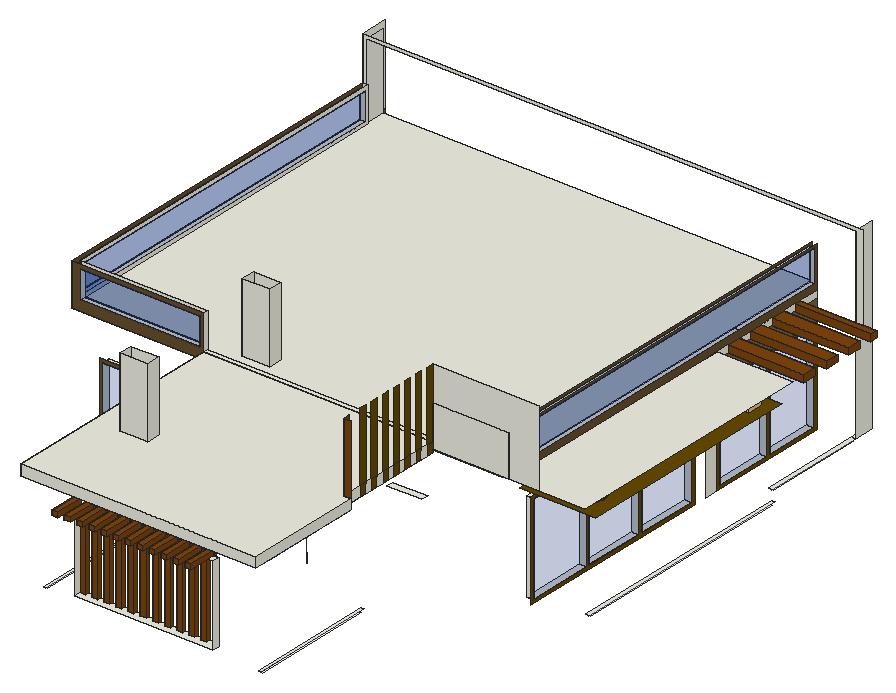
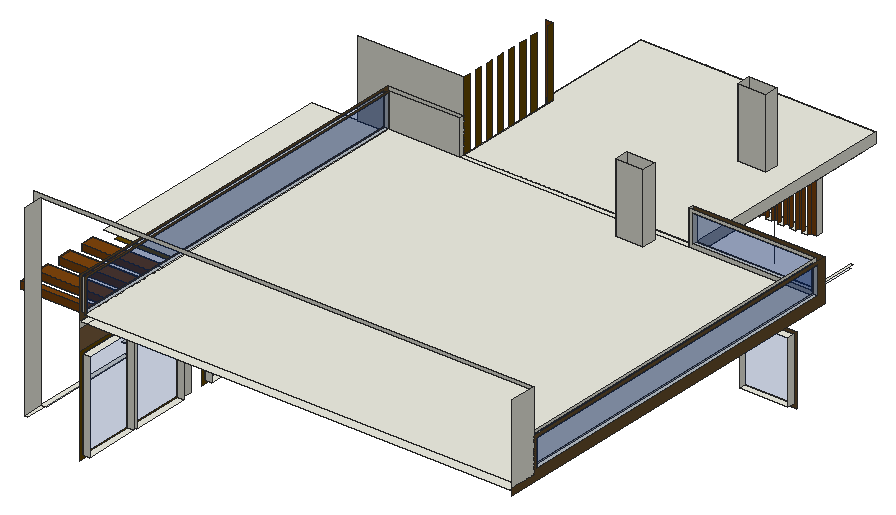
# SketchUp Ruby script. Lengths in inches.
U = 1.inch
M = Sketchup.active_model
def pt(a) = Geom::Point3d.new(a.map { |v| v * U })
def face(e, loops, mat)
  f = e.add_face(loops[0].map { |a| pt(a) })
  loops[1..].each { |l| e.add_face(l.map { |a| pt(a) }).erase! }
  f.material = f.back_material = mat if mat
  f
end
# faces: each face lists its corners as indices into pts; further lists are holes
def faces(e, pts, list, mat = nil) = list.each { |f| face(e, (f[0].is_a?(Array) ? f : [f]).map { |l| l.map { |i| pts[i] } }, mat) }
# xy, xz, yz: faces in a plane at the given z, y or x. An outline is a flat list of corners, or four numbers for a rectangle; further outlines are holes
def ring(l) = l.size == 4 ? [[l[0], l[1]], [l[2], l[1]], [l[2], l[3]], [l[0], l[3]]] : l.each_slice(2).to_a
def flat(e, list, mat, &to3) = list.each { |f| face(e, (f[0].is_a?(Array) ? f : [f]).map { |l| ring(l).map { |u, v| to3.(u, v) } }, mat) }
def xy(e, z, list, mat = nil) = flat(e, list, mat) { |x, y| [x, y, z] }
def xz(e, y, list, mat = nil) = flat(e, list, mat) { |x, z| [x, y, z] }
def yz(e, x, list, mat = nil) = flat(e, list, mat) { |y, z| [x, y, z] }
def lines(e, pts, list) = list.each { |a, b| e.add_line(pt(pts[a]), pt(pts[b])) }
# prism: a flat outline (further loops are holes) pulled along v
def prism(e, loops, v, mat = nil)
  f = face(e, loops, mat); d = Geom::Vector3d.new(v.map { |x| x * U })
  f.pushpull(f.normal.samedirection?(d) ? d.length : -d.length)
end
def box(e, o, s, mat = nil) = prism(e, [[o, [o[0] + s[0], o[1], o[2]], [o[0] + s[0], o[1] + s[1], o[2]], [o[0], o[1] + s[1], o[2]]]], [0, 0, s[2]], mat)
def at(x, y, z, deg = 0) = Geom::Transformation.translation(pt([x, y, z])) * Geom::Transformation.rotation(ORIGIN, Z_AXIS, deg.degrees)
def axes(o, x, y, z) = Geom::Transformation.new([*x, 0, *y, 0, *z, 0, *pt(o).to_a, 1])
def part(name) = M.definitions.add(name)
# library, detail: a bought-in or finely detailed component or shape, given as its bounding box
def library(name, o, s) = part(name).tap { |d| box(d.entities, o, s) }
def detail(e, o, s) = box(e.add_group.entities, o, s)
def put(e, d, t, mat = nil) = e.add_instance(d, t).tap { |i| i.material = mat if mat }
def group(e, t, mat = nil) = e.add_group.tap { |g| g.transformation = t; g.material = mat if mat }.entities
root = M.entities
M.materials.add("C08_Toffee_Ember").color = [127, 69, 12]
M.materials.add("D01_Frost_White").color = [238, 238, 227]
M.materials.add("D08_Bronzed_Mustard").color = [102, 74, 0]
M.materials.add("Glass_Basic_01").color = [161, 173, 186]
M.materials["Glass_Basic_01"].alpha = 0.25
M.materials.add("Glass_Sky Reflection_01").color = [0, 46, 142]
M.materials["Glass_Sky Reflection_01"].alpha = 0.25
M.materials.add("Plywood_01_1K").color = [125, 96, 64]
M.materials.add("Wood_Veneer_15_1K").color = [103, 79, 44]
c1 = part("Group71\#2")
p = [[0,0,0],[0,0,-29.19],[-0.46,0,-29.19],[3,-91.5,0],[-3,-91.5,0],[3,91.5,0],
  [3,0,0],[-3,91.5,0],[0.46,0,-29.19],[-3,0,0],[0,0,-47.25]]
lines(c1.entities,p,[[0,1],[1,2],[3,4],[5,6],[7,5],[1,8],[9,0],[0,6],[8,10],[4,9],[6,3],[2,10],
  [9,7]])
c2 = part("Rectangle Light")
put(c2.entities,c1,at(0,0,0))
c3 = part("Group73\#1")
p = [[0,0,0],[0,0,-14.36],[-0.46,0,-14.36],[3,-43.5,0],[-3,-43.5,0],[3,43.5,0],
  [3,0,0],[-3,43.5,0],[0.46,0,-14.36],[-3,0,0],[0,0,-23.25]]
lines(c3.entities,p,[[0,1],[1,2],[3,4],[5,6],[7,5],[1,8],[9,0],[0,6],[8,10],[4,9],[6,3],[2,10],
  [9,7]])
c4 = part("Rectangle Light\#1")
put(c4.entities,c3,at(0,0,0))
c5 = library("Sphere Light\#17",[-6.75,-6.75,-6.75],[13.5,13.5,13.5])
c6 = library("Sphere Light\#18",[-6.55,-6.55,-6.55],[13.1,13.1,13.1])
c7 = library("Sphere Light\#15",[-5.37,-5.37,-5.37],[10.74,10.74,10.74])
c8 = library("Sphere Light\#16",[-5.33,-5.33,-5.33],[10.66,10.66,10.66])
xy(root,165,[[376,388,382,445.01],[376,448.01,382,502.01],[376,505.01,382,559.02],[376,589,382,640],[376,643,382,691]],"D01_Frost_White")
xy(root,175,[[126,180,128,359],[312,180,314,287]],"Glass_Basic_01")
xy(root,177,[[126,178,128,361],[312,178,314,289]],"D01_Frost_White")
xy(root,178,[[439,375,442,572.02],[427,588,430,674]],"Glass_Basic_01")
xy(root,180,[[439,373,442,574.02],[427,586,430,676],[427,676,430,694]],"D01_Frost_White")
xy(root,183,[[31,361,73,367]],"D01_Frost_White")
xy(root,186,[[160,169,280,169,280,175,274.78,175,274.78,178,269.57,178,269.57,175,264.35,175,264.35,178,259.13,178,259.13,175,253.91,175,253.91,178,248.7,178,248.7,175,243.48,175,243.48,178,238.26,178,238.26,175,233.04,175,233.04,178,227.83,178,227.83,175,222.61,175,222.61,178,217.39,178,217.39,175,212.17,175,212.17,178,206.96,178,206.96,175,201.74,175,201.74,178,196.52,178,196.52,175,191.3,175,191.3,178,186.09,178,186.09,175,180.87,175,180.87,178,175.65,178,175.65,175,170.43,175,170.43,178,165.22,178,165.22,175,160,175]],"D01_Frost_White")
xy(root,218,[[138,361,158,367]],"D01_Frost_White")
xy(root,228,[[277,361,307,367]],"D01_Frost_White")
xy(root,237,[[31,361,73,367]],"D01_Frost_White")
xy(root,238,[[138,361,158,367]],"D01_Frost_White")
xy(root,243,[[376,388,382,445.01],[376,448.01,382,502.01],[376,505.01,382,559.02],[376,589,382,640],[376,643,382,691]],"D01_Frost_White")
xy(root,255,[[160,169,160,175,165.22,175,165.22,178,170.43,178,170.43,175,175.65,175,175.65,178,180.87,178,180.87,175,186.09,175,186.09,178,191.3,178,191.3,175,196.52,175,196.52,178,201.74,178,201.74,175,206.96,175,206.96,178,212.17,178,212.17,175,217.39,175,217.39,178,222.61,178,222.61,175,227.83,175,227.83,178,233.04,178,233.04,175,238.26,175,238.26,178,243.48,178,243.48,175,248.7,175,248.7,178,253.91,178,253.91,175,259.13,175,259.13,178,264.35,178,264.35,175,269.57,175,269.57,178,274.78,178,274.78,175,280,175,280,169]],"D01_Frost_White")
xy(root,258,[[[382,373,448,574.02],[429.95,390.2,431.52,390.3125,432.99,390.83,434.29,391.71,435.3125,392.9,435.99,394.31,436.28,395.85,436.17,397.41,435.65,398.89,434.77,400.18,433.58,401.2,432.17,401.88,430.63,402.18,429.07,402.06,427.59,401.54,426.3,400.66,425.28,399.48,424.6,398.06,424.3,396.53,424.42,394.96,424.9375,393.49,425.82,392.19,427,391.17,428.42,390.49],[388.9375,390.2,390.5,390.3125,391.98,390.83,393.27,391.71,394.3,392.9,394.98,394.31,395.27,395.85,395.15,397.41,394.64,398.89,393.75,400.18,392.57,401.2,391.16,401.88,389.62,402.18,388.06,402.06,386.58,401.54,385.28,400.66,384.26,399.48,383.58,398.06,383.29,396.53,383.4,394.96,383.92,393.49,384.8,392.19,385.99,391.17,387.4,390.49],[388.9375,551.54,390.5,551.66,391.98,552.17,393.27,553.06,394.3,554.24,394.98,555.65,395.27,557.19,395.15,558.75,394.64,560.23,393.75,561.53,392.57,562.55,391.16,563.23,389.62,563.52,388.06,563.41,386.58,562.89,385.28,562.01,384.26,560.82,383.58,559.41,383.29,557.87,383.4,556.31,383.92,554.83,384.8,553.54,385.99,552.51,387.4,551.83],[429.95,551.54,431.52,551.66,432.99,552.17,434.29,553.06,435.3125,554.24,435.99,555.65,436.28,557.19,436.17,558.75,435.65,560.23,434.77,561.53,433.58,562.55,432.17,563.23,430.63,563.52,429.07,563.41,427.59,562.89,426.3,562.01,425.28,560.82,424.6,559.41,424.3,557.87,424.42,556.31,424.9375,554.83,425.82,553.54,427,552.51,428.42,551.83]]],"D08_Bronzed_Mustard")
xy(root,259,[[160,145,165.22,169],[170.43,145,175.65,169],[180.87,145,186.09,169],[191.3,145,196.52,169],[201.74,145,206.96,169],
  [212.17,145,217.39,169],[222.61,145,227.83,169],[233.04,145,238.26,169],[243.48,145,248.7,169],[253.91,145,259.13,169],
  [264.35,145,269.57,169],[274.78,145,280,169]],"D08_Bronzed_Mustard")
xy(root,261,[[388.9375,390.2,387.4,390.49,385.99,391.17,384.8,392.19,383.92,393.49,383.4,394.96,383.29,396.53,383.58,398.06,384.26,399.48,385.28,400.66,386.58,401.54,388.06,402.06,389.62,402.18,391.16,401.88,392.57,401.2,393.75,400.18,394.64,398.89,395.15,397.41,395.27,395.85,394.98,394.31,394.3,392.9,393.27,391.71,391.98,390.83,390.5,390.3125],[429.95,390.2,428.42,390.49,427,391.17,425.82,392.19,424.9375,393.49,424.42,394.96,424.3,396.53,424.6,398.06,425.28,399.48,426.3,400.66,427.59,401.54,429.07,402.06,430.63,402.18,432.17,401.88,433.58,401.2,434.77,400.18,435.65,398.89,436.17,397.41,436.28,395.85,435.99,394.31,435.3125,392.9,434.29,391.71,432.99,390.83,431.52,390.3125],[388.9375,551.54,387.4,551.83,385.99,552.51,384.8,553.54,383.92,554.83,383.4,556.31,383.29,557.87,383.58,559.41,384.26,560.82,385.28,562.01,386.58,562.89,388.06,563.41,389.62,563.52,391.16,563.23,392.57,562.55,393.75,561.53,394.64,560.23,395.15,558.75,395.27,557.19,394.98,555.65,394.3,554.24,393.27,553.06,391.98,552.17,390.5,551.66],[429.95,551.54,428.42,551.83,427,552.51,425.82,553.54,424.9375,554.83,424.42,556.31,424.3,557.87,424.6,559.41,425.28,560.82,426.3,562.01,427.59,562.89,429.07,563.41,430.63,563.52,432.17,563.23,433.58,562.55,434.77,561.53,435.65,560.23,436.17,558.75,436.28,557.19,435.99,555.65,435.3125,554.24,434.29,553.06,432.99,552.17,431.52,551.66]],"D08_Bronzed_Mustard")
xy(root,263,[[160,145,165.22,169],[170.43,145,175.65,169],[180.87,145,186.09,169],[191.3,145,196.52,169],[201.74,145,206.96,169],
  [212.17,145,217.39,169],[222.61,145,227.83,169],[233.04,145,238.26,169],[243.48,145,248.7,169],[253.91,145,259.13,169],
  [264.35,145,269.57,169],[274.78,145,280,169]],"C08_Toffee_Ember")
xy(root,264,[[382,598,448,610],[382,622,448,634],[382,646,448,658],[382,670,448,676.01]],"C08_Toffee_Ember")
xy(root,267,[[118,163,118,361,316,361,316,178,322,178,322,163],[124,169,124,178,322,178,322,265,316,265,316,169],[316,178,322,265]],"D01_Frost_White")
xy(root,270,[[382,598,448,610],[382,622,448,634],[382,646,448,658],[382,670,448,670,448,676.01,436,676.01,436,676,430,676,430,676.01,382,676.01]],"C08_Toffee_Ember")
xy(root,270,[[124,169,316,178],[4,361,10,694],[10,361,376,367],[376,361,382,694],[382,361,448,586],
  [10,367,376,694],[430,676,436,676.01]],"D01_Frost_White")
xy(root,276,[[[118,163,322,163,322,265,316,265,316,361,118,361],[142,241,166,253]],[118,361,316,365.5],[[8.5,365.5,377.5,365.5,377.5,694,7,694,7,676.01,8.5,676.01],[142,373,166,385]],[377.5,365.5,382,610],[377.5,610,382,692]],"D01_Frost_White")
xy(root,279,[[11.5,361,115,365.5],[4,368.5,8.5,673.01]],"D01_Frost_White")
xz(root,145,[[160,259,165.22,263],[170.43,259,175.65,263],[180.87,259,186.09,263],[191.3,259,196.52,263],[201.74,259,206.96,263],
  [212.17,259,217.39,263],[222.61,259,227.83,263],[233.04,259,238.26,263],[243.48,259,248.7,263],[253.91,259,259.13,263],
  [264.35,259,269.57,263],[274.78,259,280,263]],"C08_Toffee_Ember")
xz(root,163,[[118,267,322,276]],"D01_Frost_White")
xz(root,169,[[124,267,316,270]],"D01_Frost_White")
xz(root,175,[[160,186,165.22,255],[170.43,186,175.65,255],[180.87,186,186.09,255],[191.3,186,196.52,255],[201.74,186,206.96,255],
  [212.17,186,217.39,255],[222.61,186,227.83,255],[233.04,186,238.26,255],[243.48,186,248.7,255],[253.91,186,259.13,255],
  [264.35,186,269.57,255],[274.78,186,280,255]],"C08_Toffee_Ember")
xz(root,178,[[124,267,316,270]],"D01_Frost_White")
xz(root,241,[[142,276,166,336]],"D01_Frost_White")
xz(root,253,[[142,276,166,336]],"D01_Frost_White")
xz(root,265,[[316,276,322,336]],"C08_Toffee_Ember")
xz(root,265,[[316,267,322,276]],"D08_Bronzed_Mustard")
xz(root,361,[[118,267,316,270],[118,270,316,276],[316,270,382,306],[382,270,382,306,316,306,316,336,408,336,408,270]],"D01_Frost_White")
xz(root,361,[[31,183,73,237],[138,218,158,238],[11.5,279,115,303]],"Glass_Sky Reflection_01")
xz(root,361,[[[28,180,76,240],[31,183,73,237]],[[136,216,160,240],[138,218,158,238]],[[4,270,118,306],[11.5,279,115,303]]],"Wood_Veneer_15_1K")
xz(root,365.5,[[[8.5,276,118,306],[11.5,279,115,303]],[316,276,377.5,306],[377.5,276,382,304]],"D01_Frost_White")
xz(root,365.5,[[11.5,279,115,303]],"Glass_Sky Reflection_01")
xz(root,368.5,[[4,279,8.5,303]],"D01_Frost_White")
xz(root,373,[[142,276,166,336]],"D01_Frost_White")
xz(root,385,[[142,276,166,336]],"D01_Frost_White")
xz(root,388,[[376,165,382,243]],"D01_Frost_White")
xz(root,445.01,[[376,165,382,243]],"D01_Frost_White")
xz(root,448.01,[[376,165,382,243]],"D01_Frost_White")
xz(root,502.01,[[376,165,382,243]],"D01_Frost_White")
xz(root,505.01,[[376,165,382,243]],"D01_Frost_White")
xz(root,559.02,[[376,165,382,243]],"D01_Frost_White")
xz(root,589,[[376,165,382,243]],"D01_Frost_White")
xz(root,598,[[382,264,448,270]],"C08_Toffee_Ember")
xz(root,610,[[382,264,448,270]],"C08_Toffee_Ember")
xz(root,622,[[382,264,448,270]],"C08_Toffee_Ember")
xz(root,634,[[382,264,448,270]],"C08_Toffee_Ember")
xz(root,640,[[376,165,382,243]],"D01_Frost_White")
xz(root,643,[[376,165,382,243]],"D01_Frost_White")
xz(root,646,[[382,264,448,270]],"C08_Toffee_Ember")
xz(root,658,[[382,264,448,270]],"C08_Toffee_Ember")
xz(root,670,[[382,264,448,270]],"C08_Toffee_Ember")
xz(root,673.01,[[4,279,8.5,303]],"D01_Frost_White")
xz(root,676.01,[[382,264,448,270]],"C08_Toffee_Ember")
xz(root,676.01,[[430,270,436,270,436,344,4,344,4,306,7,306,7,341,430,341],[7,276,8.5,306]],"D01_Frost_White")
xz(root,691,[[376,165,382,243]],"D01_Frost_White")
xz(root,692,[[377.5,276,382,304]],"D01_Frost_White")
yz(root,4,[[676.01,276,700,344]],"D01_Frost_White")
yz(root,4,[[368.5,279,673.01,303]],"Glass_Sky Reflection_01")
yz(root,4,[[[361,270,361,306,676.01,306,676.01,276,700,276,700,270],[368.5,279,673.01,303]]],"Wood_Veneer_15_1K")
yz(root,7,[[676.01,276,694,341]],"D01_Frost_White")
yz(root,8.5,[[[365.5,276,676.01,306],[368.5,279,673.01,303]]],"D01_Frost_White")
yz(root,8.5,[[368.5,279,673.01,303]],"Glass_Sky Reflection_01")
yz(root,11.5,[[361,279,365.5,303]],"D01_Frost_White")
yz(root,31,[[361,183,367,237]],"D01_Frost_White")
yz(root,73,[[361,183,367,237]],"D01_Frost_White")
yz(root,115,[[361,279,365.5,303]],"D01_Frost_White")
yz(root,118,[[163,267,361,276],[361,276,365.5,306]],"D01_Frost_White")
yz(root,124,[[169,267,178,270]],"D01_Frost_White")
yz(root,138,[[361,218,367,238]],"D01_Frost_White")
yz(root,142,[[241,276,253,336],[373,276,385,336]],"D01_Frost_White")
yz(root,158,[[361,218,367,238]],"D01_Frost_White")
yz(root,160,[[145,259,169,263]],"C08_Toffee_Ember")
yz(root,160,[[169,186,175,255]],"D01_Frost_White")
yz(root,165.22,[[175,186,178,255],[145,259,169,263]],"C08_Toffee_Ember")
yz(root,166,[[241,276,253,336],[373,276,385,336]],"D01_Frost_White")
yz(root,170.43,[[175,186,178,255],[145,259,169,263]],"C08_Toffee_Ember")
yz(root,175.65,[[175,186,178,255],[145,259,169,263]],"C08_Toffee_Ember")
yz(root,180.87,[[175,186,178,255],[145,259,169,263]],"C08_Toffee_Ember")
yz(root,186.09,[[175,186,178,255],[145,259,169,263]],"C08_Toffee_Ember")
yz(root,191.3,[[175,186,178,255],[145,259,169,263]],"C08_Toffee_Ember")
yz(root,196.52,[[175,186,178,255],[145,259,169,263]],"C08_Toffee_Ember")
yz(root,201.74,[[175,186,178,255],[145,259,169,263]],"C08_Toffee_Ember")
yz(root,206.96,[[175,186,178,255],[145,259,169,263]],"C08_Toffee_Ember")
yz(root,212.17,[[175,186,178,255],[145,259,169,263]],"C08_Toffee_Ember")
yz(root,217.39,[[175,186,178,255],[145,259,169,263]],"C08_Toffee_Ember")
yz(root,222.61,[[175,186,178,255],[145,259,169,263]],"C08_Toffee_Ember")
yz(root,227.83,[[175,186,178,255],[145,259,169,263]],"C08_Toffee_Ember")
yz(root,233.04,[[175,186,178,255],[145,259,169,263]],"C08_Toffee_Ember")
yz(root,238.26,[[175,186,178,255],[145,259,169,263]],"C08_Toffee_Ember")
yz(root,243.48,[[175,186,178,255],[145,259,169,263]],"C08_Toffee_Ember")
yz(root,248.7,[[175,186,178,255],[145,259,169,263]],"C08_Toffee_Ember")
yz(root,253.91,[[175,186,178,255],[145,259,169,263]],"C08_Toffee_Ember")
yz(root,259.13,[[175,186,178,255],[145,259,169,263]],"C08_Toffee_Ember")
yz(root,264.35,[[175,186,178,255],[145,259,169,263]],"C08_Toffee_Ember")
yz(root,269.57,[[175,186,178,255],[145,259,169,263]],"C08_Toffee_Ember")
yz(root,274.78,[[175,186,178,255],[145,259,169,263]],"C08_Toffee_Ember")
yz(root,280,[[145,259,169,263]],"C08_Toffee_Ember")
yz(root,280,[[169,186,175,255]],"D01_Frost_White")
yz(root,316,[[169,267,178,270],[271,267,283,276],[289,267,295,276],[301,267,307,276],[313,267,319,276],
  [325,267,331,276],[337,267,343,276],[349,267,355,276],[361,276,365.5,306]],"D01_Frost_White")
yz(root,316,[[265,267,271,276],[283,267,289,276],[295,267,301,276],[307,267,313,276],[319,267,325,276],
  [331,267,337,276],[343,267,349,276],[355,267,361,276],[265,276,271,336],[283,276,289,336],
  [295,276,301,336],[307,276,313,336],[319,276,325,336],[331,276,337,336],[343,276,349,336],
  [355,276,361,336]],"D08_Bronzed_Mustard")
yz(root,322,[[163,267,265,276]],"D01_Frost_White")
yz(root,377.5,[[365.5,276,692,304]],"Glass_Sky Reflection_01")
yz(root,377.5,[[692,276,692,304,365.5,304,365.5,306,694,306,694,276]],"Wood_Veneer_15_1K")
yz(root,382,[[574.02,162,586,246],[574.02,246,586,270],[586,264,598,270],[610,264,622,270],[634,264,646,270],
  [658,264,670,270],[676.01,264,694,270]],"D01_Frost_White")
yz(root,382,[[[385,162,562.02,246],[388,165,388,243,445.01,243,445.01,165,448.01,165,448.01,243,502.01,243,502.01,165,505.01,165,505.01,243,559.02,243,559.02,165]],[[586,162,694,246],[589,165,589,243,640,243,640,165,643,165,643,243,691,243,691,165]]],"D08_Bronzed_Mustard")
yz(root,382,[[388,165,445.01,243],[448.01,165,502.01,243],[505.01,165,559.02,243],[589,165,640,243],[643,165,691,243],
  [365.5,276,692,304]],"Glass_Sky Reflection_01")
yz(root,382,[[586,246,694,264]],"Plywood_01_1K")
yz(root,382,[[[361,270,694,306],[365.5,276,692,304]]],"Wood_Veneer_15_1K")
yz(root,430,[[676,180,676,270,676.01,270,676.01,341,694,341,694,180]],"D01_Frost_White")
yz(root,448,[[598,264,610,270],[622,264,634,270],[646,264,658,270],[670,264,676.01,270]],"C08_Toffee_Ember")
p = [[388.9375,390.2,258],[387.4,390.49,258],[387.4,390.49,261],[388.9375,390.2,261],[390.5,390.3125,258],[390.5,390.3125,261],
  [429.95,390.2,258],[428.42,390.49,258],[428.42,390.49,261],[429.95,390.2,261],[431.52,390.3125,258],[431.52,390.3125,261],
  [391.98,390.83,258],[391.98,390.83,261],[432.99,390.83,258],[432.99,390.83,261],[385.99,391.17,258],[385.99,391.17,261],
  [427,391.17,258],[427,391.17,261],[393.27,391.71,258],[393.27,391.71,261],[434.29,391.71,258],[434.29,391.71,261],
  [384.8,392.19,258],[384.8,392.19,261],[425.82,392.19,258],[425.82,392.19,261],[394.3,392.9,258],[394.3,392.9,261],
  [435.3125,392.9,258],[435.3125,392.9,261],[383.92,393.49,258],[383.92,393.49,261],[424.9375,393.49,258],[424.9375,393.49,261],
  [394.98,394.31,258],[394.98,394.31,261],[435.99,394.31,258],[435.99,394.31,261],[383.4,394.96,258],[383.4,394.96,261],
  [424.42,394.96,258],[424.42,394.96,261],[395.27,395.85,258],[395.27,395.85,261],[436.28,395.85,258],[436.28,395.85,261],
  [383.29,396.53,258],[383.29,396.53,261],[424.3,396.53,258],[424.3,396.53,261],[395.15,397.41,258],[395.15,397.41,261],
  [436.17,397.41,258],[436.17,397.41,261],[383.58,398.06,258],[383.58,398.06,261],[424.6,398.06,258],[424.6,398.06,261],
  [394.64,398.89,258],[394.64,398.89,261],[435.65,398.89,258],[435.65,398.89,261],[384.26,399.48,258],[384.26,399.48,261],
  [425.28,399.48,258],[425.28,399.48,261],[393.75,400.18,258],[393.75,400.18,261],[434.77,400.18,258],[434.77,400.18,261],
  [385.28,400.66,258],[385.28,400.66,261],[426.3,400.66,258],[426.3,400.66,261],[392.57,401.2,258],[392.57,401.2,261],
  [433.58,401.2,258],[433.58,401.2,261],[386.58,401.54,258],[386.58,401.54,261],[427.59,401.54,258],[427.59,401.54,261],
  [391.16,401.88,258],[391.16,401.88,261],[432.17,401.88,258],[432.17,401.88,261],[388.06,402.06,258],[388.06,402.06,261],
  [429.07,402.06,258],[429.07,402.06,261],[389.62,402.18,258],[389.62,402.18,261],[430.63,402.18,258],[430.63,402.18,261],
  [388.9375,551.54,258],[387.4,551.83,258],[387.4,551.83,261],[388.9375,551.54,261],[390.5,551.66,258],[390.5,551.66,261],
  [429.95,551.54,258],[428.42,551.83,258],[428.42,551.83,261],[429.95,551.54,261],[431.52,551.66,258],[431.52,551.66,261],
  [391.98,552.17,258],[391.98,552.17,261],[432.99,552.17,258],[432.99,552.17,261],[385.99,552.51,258],[385.99,552.51,261],
  [427,552.51,258],[427,552.51,261],[393.27,553.06,258],[393.27,553.06,261],[434.29,553.06,258],[434.29,553.06,261],
  [384.8,553.54,258],[384.8,553.54,261],[425.82,553.54,258],[425.82,553.54,261],[394.3,554.24,258],[394.3,554.24,261],
  [435.3125,554.24,258],[435.3125,554.24,261],[383.92,554.83,258],[383.92,554.83,261],[424.9375,554.83,258],[424.9375,554.83,261],
  [394.98,555.65,258],[394.98,555.65,261],[435.99,555.65,258],[435.99,555.65,261],[383.4,556.31,258],[383.4,556.31,261],
  [424.42,556.31,258],[424.42,556.31,261],[395.27,557.19,258],[395.27,557.19,261],[436.28,557.19,258],[436.28,557.19,261],
  [383.29,557.87,258],[383.29,557.87,261],[424.3,557.87,258],[424.3,557.87,261],[395.15,558.75,258],[395.15,558.75,261],
  [436.17,558.75,258],[436.17,558.75,261],[383.58,559.41,258],[383.58,559.41,261],[424.6,559.41,258],[424.6,559.41,261],
  [394.64,560.23,258],[394.64,560.23,261],[435.65,560.23,258],[435.65,560.23,261],[384.26,560.82,258],[384.26,560.82,261],
  [425.28,560.82,258],[425.28,560.82,261],[393.75,561.53,258],[393.75,561.53,261],[434.77,561.53,258],[434.77,561.53,261],
  [385.28,562.01,258],[385.28,562.01,261],[426.3,562.01,258],[426.3,562.01,261],[392.57,562.55,258],[392.57,562.55,261],
  [433.58,562.55,258],[433.58,562.55,261],[386.58,562.89,258],[386.58,562.89,261],[427.59,562.89,258],[427.59,562.89,261],
  [391.16,563.23,258],[391.16,563.23,261],[432.17,563.23,258],[432.17,563.23,261],[388.06,563.41,258],[388.06,563.41,261],
  [429.07,563.41,258],[429.07,563.41,261],[389.62,563.52,258],[389.62,563.52,261],[430.63,563.52,258],[430.63,563.52,261],
  [280,169,263],[160,175,255],[274.78,169,263],[269.57,169,263],[264.35,169,263],[259.13,169,263],
  [253.91,169,263],[248.7,169,263],[243.48,169,263],[238.26,169,263],[233.04,169,263],[227.83,169,263],
  [222.61,169,263],[217.39,169,263],[212.17,169,263],[206.96,169,263],[201.74,169,263],[196.52,169,263],
  [191.3,169,263],[186.09,169,263],[180.87,169,263],[175.65,169,263],[170.43,169,263],[165.22,169,263]]
faces(root,p,[[0,1,2,3],[4,0,3,5],[6,7,8,9],[10,6,9,11],[12,4,5,13],[14,10,11,15],[1,16,17,2],[7,18,19,8],
  [20,12,13,21],[22,14,15,23],[16,24,25,17],[18,26,27,19],[28,20,21,29],[30,22,23,31],[24,32,33,25],[26,34,35,27],
  [36,28,29,37],[38,30,31,39],[32,40,41,33],[34,42,43,35],[44,36,37,45],[46,38,39,47],[40,48,49,41],[42,50,51,43],
  [52,44,45,53],[54,46,47,55],[48,56,57,49],[50,58,59,51],[60,52,53,61],[62,54,55,63],[56,64,65,57],[58,66,67,59],
  [68,60,61,69],[70,62,63,71],[64,72,73,65],[66,74,75,67],[76,68,69,77],[78,70,71,79],[72,80,81,73],[74,82,83,75],
  [84,76,77,85],[86,78,79,87],[80,88,89,81],[82,90,91,83],[92,84,85,93],[94,86,87,95],[88,92,93,89],[90,94,95,91],
  [96,97,98,99],[100,96,99,101],[102,103,104,105],[106,102,105,107],[108,100,101,109],[110,106,107,111],[97,112,113,98],[103,114,115,104],
  [116,108,109,117],[118,110,111,119],[112,120,121,113],[114,122,123,115],[124,116,117,125],[126,118,119,127],[120,128,129,121],[122,130,131,123],
  [132,124,125,133],[134,126,127,135],[128,136,137,129],[130,138,139,131],[140,132,133,141],[142,134,135,143],[136,144,145,137],[138,146,147,139],
  [148,140,141,149],[150,142,143,151],[144,152,153,145],[146,154,155,147],[156,148,149,157],[158,150,151,159],[152,160,161,153],[154,162,163,155],
  [164,156,157,165],[166,158,159,167],[160,168,169,161],[162,170,171,163],[172,164,165,173],[174,166,167,175],[168,176,177,169],[170,178,179,171],
  [180,172,173,181],[182,174,175,183],[176,184,185,177],[178,186,187,179],[188,180,181,189],[190,182,183,191],[184,188,189,185],[186,190,191,187]],"D08_Bronzed_Mustard")
lines(root,p,[[192,193],[194,195],[196,197],[198,199],[200,201],[202,203],[204,205],[206,207],[208,209],[210,211],[212,213],[214,215]])
put(root,c2,axes([121,269.5,266.99],[-1,0,0],[0,1,0],[0,0,1]),"D01_Frost_White")
put(root,c4,axes([319,221.5,266.99],[-1,0,0],[0,1,0],[0,0,1]),"D01_Frost_White")
put(root,c5,at(431.02,557.36,261),"D01_Frost_White")
put(root,c6,at(389.83,557.46,261),"D01_Frost_White")
put(root,c7,at(429.65,396.05,261),"D01_Frost_White")
put(root,c8,at(389.02,396.08,261),"D01_Frost_White")
